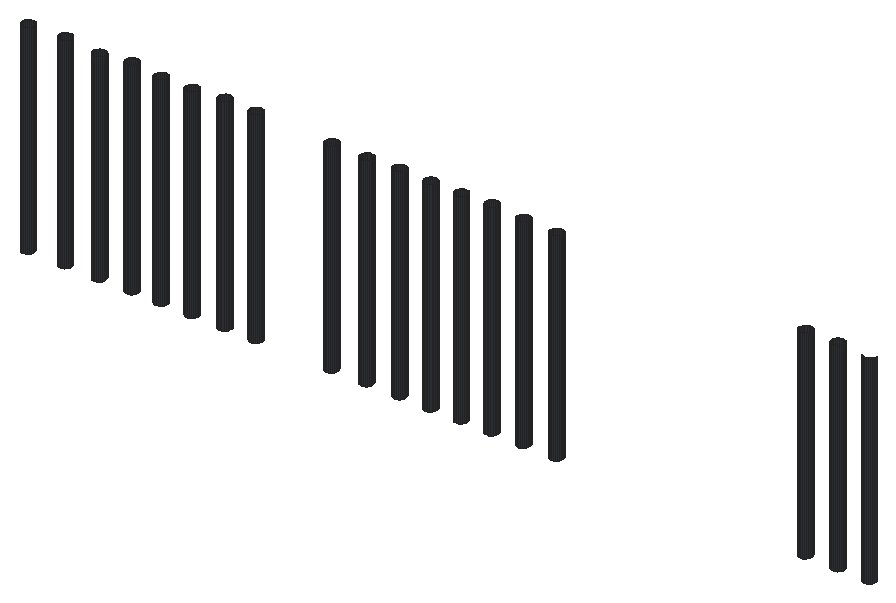
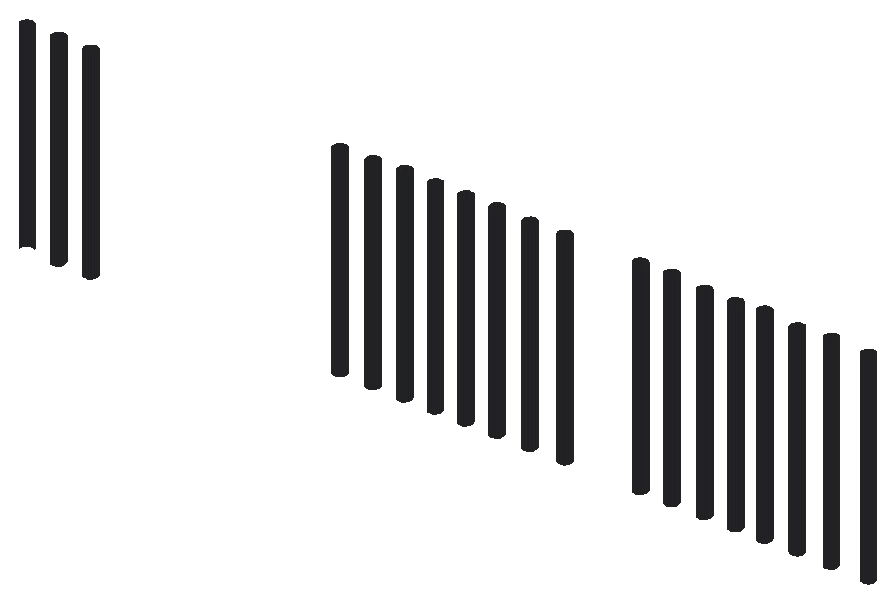
# SketchUp Ruby script. Lengths in inches.
U = 1.inch
M = Sketchup.active_model
def pt(a) = Geom::Point3d.new(a.map { |v| v * U })
def face(e, loops, mat)
  f = e.add_face(loops[0].map { |a| pt(a) })
  loops[1..].each { |l| e.add_face(l.map { |a| pt(a) }).erase! }
  f.material = f.back_material = mat if mat
  f
end
# faces: each face lists its corners as indices into pts; further lists are holes
def faces(e, pts, list, mat = nil) = list.each { |f| face(e, (f[0].is_a?(Array) ? f : [f]).map { |l| l.map { |i| pts[i] } }, mat) }
# xy, xz, yz: faces in a plane at the given z, y or x. An outline is a flat list of corners, or four numbers for a rectangle; further outlines are holes
def ring(l) = l.size == 4 ? [[l[0], l[1]], [l[2], l[1]], [l[2], l[3]], [l[0], l[3]]] : l.each_slice(2).to_a
def flat(e, list, mat, &to3) = list.each { |f| face(e, (f[0].is_a?(Array) ? f : [f]).map { |l| ring(l).map { |u, v| to3.(u, v) } }, mat) }
def xy(e, z, list, mat = nil) = flat(e, list, mat) { |x, y| [x, y, z] }
def xz(e, y, list, mat = nil) = flat(e, list, mat) { |x, z| [x, y, z] }
def yz(e, x, list, mat = nil) = flat(e, list, mat) { |y, z| [x, y, z] }
def lines(e, pts, list) = list.each { |a, b| e.add_line(pt(pts[a]), pt(pts[b])) }
# prism: a flat outline (further loops are holes) pulled along v
def prism(e, loops, v, mat = nil)
  f = face(e, loops, mat); d = Geom::Vector3d.new(v.map { |x| x * U })
  f.pushpull(f.normal.samedirection?(d) ? d.length : -d.length)
end
def box(e, o, s, mat = nil) = prism(e, [[o, [o[0] + s[0], o[1], o[2]], [o[0] + s[0], o[1] + s[1], o[2]], [o[0], o[1] + s[1], o[2]]]], [0, 0, s[2]], mat)
def at(x, y, z, deg = 0) = Geom::Transformation.translation(pt([x, y, z])) * Geom::Transformation.rotation(ORIGIN, Z_AXIS, deg.degrees)
def axes(o, x, y, z) = Geom::Transformation.new([*x, 0, *y, 0, *z, 0, *pt(o).to_a, 1])
def part(name) = M.definitions.add(name)
# library, detail: a bought-in or finely detailed component or shape, given as its bounding box
def library(name, o, s) = part(name).tap { |d| box(d.entities, o, s) }
def detail(e, o, s) = box(e.add_group.entities, o, s)
def put(e, d, t, mat = nil) = e.add_instance(d, t).tap { |i| i.material = mat if mat }
def group(e, t, mat = nil) = e.add_group.tap { |g| g.transformation = t; g.material = mat if mat }.entities
root = M.entities
M.materials.add("[Formica Laminate Dark]1").color = [50, 53, 60]
xy(root,29.875,[[1934.18,55.58,1931.67,55.72,1929.29,56.51,1927.18,57.89,1925.51,59.76,1924.38,62.01,1923.87,64.47,1924.01,66.98,1924.8,69.36,1926.18,71.46,1928.05,73.14,1930.29,74.27,1932.75,74.78,1935.26,74.64,1937.65,73.85,1939.75,72.47,1941.42,70.6,1942.55,68.35,1943.07,65.89,1942.92,63.38,1942.14,61,1940.76,58.9,1938.88,57.22,1936.64,56.09],[1991.49,55.58,1988.98,55.72,1986.6,56.51,1984.5,57.89,1982.82,59.76,1981.69,62.01,1981.18,64.47,1981.32,66.98,1982.11,69.36,1983.49,71.46,1985.36,73.14,1987.61,74.27,1990.07,74.78,1992.58,74.64,1994.96,73.85,1997.0625,72.47,1998.74,70.6,1999.87,68.35,2000.38,65.89,2000.24,63.38,1999.45,61,1998.07,58.9,1996.2,57.22,1993.95,56.09],[2044.37,55.58,2041.86,55.72,2039.47,56.51,2037.37,57.89,2035.7,59.76,2034.57,62.01,2034.06,64.47,2034.2,66.98,2034.99,69.36,2036.36,71.46,2038.24,73.14,2040.48,74.27,2042.94,74.78,2045.45,74.64,2047.84,73.85,2049.9375,72.47,2051.61,70.6,2052.74,68.35,2053.25,65.89,2053.11,63.38,2052.32,61,2050.95,58.9,2049.07,57.22,2046.83,56.09],[2094.55,55.58,2092.05,55.72,2089.66,56.51,2087.56,57.89,2085.89,59.76,2084.76,62.01,2084.24,64.47,2084.39,66.98,2085.17,69.36,2086.55,71.46,2088.43,73.14,2090.67,74.27,2093.13,74.78,2095.64,74.64,2098.02,73.85,2100.125,72.47,2101.8,70.6,2102.93,68.35,2103.44,65.89,2103.3,63.38,2102.51,61,2101.13,58.9,2099.26,57.22,2097.01,56.09],[2404.12,55.58,2401.61,55.72,2399.22,56.51,2397.12,57.89,2395.45,59.76,2394.32,62.01,2393.81,64.47,2393.95,66.98,2394.74,69.36,2396.11,71.46,2397.99,73.14,2400.23,74.27,2402.69,74.78,2405.2,74.64,2407.59,73.85,2409.6875,72.47,2411.36,70.6,2412.49,68.35,2413,65.89,2412.86,63.38,2412.07,61,2410.7,58.9,2408.82,57.22,2406.58,56.09],
  [2458.12,55.58,2455.61,55.72,2453.22,56.51,2451.12,57.89,2449.45,59.76,2448.32,62.01,2447.81,64.47,2447.95,66.98,2448.74,69.36,2450.11,71.46,2451.99,73.14,2454.23,74.27,2456.69,74.78,2459.2,74.64,2461.59,73.85,2463.6875,72.47,2465.36,70.6,2466.49,68.35,2467,65.89,2466.86,63.38,2466.07,61,2464.7,58.9,2462.82,57.22,2460.58,56.09],[2604.55,55.58,2602.05,55.72,2599.66,56.51,2597.56,57.89,2595.89,59.76,2594.76,62.01,2594.24,64.47,2594.39,66.98,2595.17,69.36,2596.55,71.46,2598.43,73.14,2600.67,74.27,2603.13,74.78,2605.64,74.64,2608.02,73.85,2610.125,72.47,2611.8,70.6,2612.93,68.35,2613.44,65.89,2613.3,63.38,2612.51,61,2611.13,58.9,2609.26,57.22,2607.01,56.09],[2700.93,55.58,2698.42,55.72,2696.04,56.51,2693.93,57.89,2692.26,59.76,2691.13,62.01,2690.62,64.47,2690.76,66.98,2691.55,69.36,2692.93,71.46,2694.8,73.14,2697.04,74.27,2699.5,74.78,2702.01,74.64,2704.4,73.85,2706.5,72.47,2708.17,70.6,2709.3,68.35,2709.82,65.89,2709.67,63.38,2708.89,61,2707.51,58.9,2705.63,57.22,2703.39,56.09],[2752.12,55.58,2749.61,55.72,2747.22,56.51,2745.12,57.89,2743.45,59.76,2742.32,62.01,2741.81,64.47,2741.95,66.98,2742.74,69.36,2744.11,71.46,2745.99,73.14,2748.23,74.27,2750.69,74.78,2753.2,74.64,2755.59,73.85,2757.6875,72.47,2759.36,70.6,2760.49,68.35,2761,65.89,2760.86,63.38,2760.07,61,2758.7,58.9,2756.82,57.22,2754.58,56.09]])
p = [[1931.67,55.72,29.875],[1934.18,55.58,29.875],[1934.18,55.58,343.5],[1931.67,55.72,343.5],[1936.64,56.09,29.875],[1936.64,56.09,343.5],
  [1988.98,55.72,29.875],[1991.49,55.58,29.875],[1991.49,55.58,345.54],[1988.98,55.72,345.54],[1993.95,56.09,29.875],[1993.95,56.09,345.54],
  [2041.86,55.72,29.875],[2044.37,55.58,29.875],[2044.37,55.58,341.4375],[2041.86,55.72,341.4375],[2046.83,56.09,29.875],[2046.83,56.09,341.4375],
  [2092.05,55.72,29.875],[2094.55,55.58,29.875],[2094.55,55.58,347.25],[2092.05,55.72,347.25],[2097.01,56.09,29.875],[2097.01,56.09,347.25],
  [2137.48,55.72,29.875],[2139.99,55.58,29.875],[2139.99,55.58,342.8],[2137.48,55.72,342.8],[2142.45,56.09,29.875],[2142.45,56.09,342.8],
  [2185.48,55.72,29.875],[2187.99,55.58,29.875],[2187.99,55.58,343.0625],[2185.48,55.72,343.0625],[2190.45,56.09,29.875],[2190.45,56.09,343.0625],
  [2236.17,55.72,29.875],[2238.68,55.58,29.875],[2238.68,55.58,347.3125],[2236.17,55.72,347.3125],[2241.14,56.09,29.875],[2241.14,56.09,347.3125],
  [2284.48,55.72,29.875],[2286.99,55.58,29.875],[2286.99,55.58,346.125],[2284.48,55.72,346.125],[2289.45,56.09,29.875],[2289.45,56.09,346.125],
  [2401.61,55.72,29.875],[2404.12,55.58,29.875],[2404.12,55.58,343.625],[2401.61,55.72,343.625],[2406.58,56.09,29.875],[2406.58,56.09,343.625],
  [2455.61,55.72,29.875],[2458.12,55.58,29.875],[2458.12,55.58,342.8],[2455.61,55.72,342.8],[2460.58,56.09,29.875],[2460.58,56.09,342.8],
  [2506.42,55.72,29.875],[2508.93,55.58,29.875],[2508.93,55.58,345],[2506.42,55.72,345],[2511.39,56.09,29.875],[2511.39,56.09,345],
  [2554.98,55.72,29.875],[2557.49,55.58,29.875],[2557.49,55.58,344.25],[2554.98,55.72,344.25],[2559.95,56.09,29.875],[2559.95,56.09,344.25],
  [2602.05,55.72,29.875],[2604.55,55.58,29.875],[2604.55,55.58,344.375],[2602.05,55.72,344.375],[2607.01,56.09,29.875],[2607.01,56.09,344.375],
  [2649.42,55.72,29.875],[2651.93,55.58,29.875],[2651.93,55.58,346],[2649.42,55.72,346],[2654.39,56.09,29.875],[2654.39,56.09,346],
  [2698.42,55.72,29.875],[2700.93,55.58,29.875],[2700.93,55.58,342.8],[2698.42,55.72,342.8],[2703.39,56.09,29.875],[2703.39,56.09,342.8],
  [2749.61,55.72,29.875],[2752.12,55.58,29.875],[2752.12,55.58,341.625],[2749.61,55.72,341.625],[2754.58,56.09,29.875],[2754.58,56.09,341.625],
  [3135.36,55.72,29.875],[3137.87,55.58,29.875],[3137.87,55.58,342.54],[3135.36,55.72,342.54],[3140.33,56.09,29.875],[3140.33,56.09,342.54],
  [3185.48,55.72,29.875],[3187.99,55.58,29.875],[3187.99,55.58,342.54],[3185.48,55.72,342.54],[3190.45,56.09,29.875],[3190.45,56.09,342.54],
  [3234.42,55.72,29.875],[3236.93,55.58,29.875],[3236.93,55.58,342.54],[3234.42,55.72,342.54],[3239.39,56.09,29.875],[3239.39,56.09,342.54],
  [1929.29,56.51,29.875],[1929.29,56.51,343.5],[1986.6,56.51,29.875],[1986.6,56.51,345.54],[2039.47,56.51,29.875],[2039.47,56.51,341.4375],
  [2089.66,56.51,29.875],[2089.66,56.51,347.25],[2135.1,56.51,29.875],[2135.1,56.51,342.8],[2183.1,56.51,29.875],[2183.1,56.51,343.0625],
  [2233.79,56.51,29.875],[2233.79,56.51,347.3125],[2282.1,56.51,29.875],[2282.1,56.51,346.125],[2399.22,56.51,29.875],[2399.22,56.51,343.625],
  [2453.22,56.51,29.875],[2453.22,56.51,342.8],[2504.04,56.51,29.875],[2504.04,56.51,345],[2552.6,56.51,29.875],[2552.6,56.51,344.25],
  [2599.66,56.51,29.875],[2599.66,56.51,344.375],[2647.04,56.51,29.875],[2647.04,56.51,346],[2696.04,56.51,29.875],[2696.04,56.51,342.8],
  [2747.22,56.51,29.875],[2747.22,56.51,341.625],[3132.97,56.51,29.875],[3132.97,56.51,342.54],[3183.1,56.51,29.875],[3183.1,56.51,342.54],
  [3232.04,56.51,29.875],[3232.04,56.51,342.54],[1938.88,57.22,29.875],[1938.88,57.22,343.5],[1996.2,57.22,29.875],[1996.2,57.22,345.54],
  [2049.07,57.22,29.875],[2049.07,57.22,341.4375],[2099.26,57.22,29.875],[2099.26,57.22,347.25],[2144.7,57.22,29.875],[2144.7,57.22,342.8],
  [2192.7,57.22,29.875],[2192.7,57.22,343.0625],[2243.38,57.22,29.875],[2243.38,57.22,347.3125],[2291.7,57.22,29.875],[2291.7,57.22,346.125],
  [2408.82,57.22,29.875],[2408.82,57.22,343.625],[2462.82,57.22,29.875],[2462.82,57.22,342.8],[2513.63,57.22,29.875],[2513.63,57.22,345],
  [2562.2,57.22,29.875],[2562.2,57.22,344.25],[2609.26,57.22,29.875],[2609.26,57.22,344.375],[2656.63,57.22,29.875],[2656.63,57.22,346],
  [2705.63,57.22,29.875],[2705.63,57.22,342.8],[2756.82,57.22,29.875],[2756.82,57.22,341.625],[3142.57,57.22,29.875],[3142.57,57.22,342.54],
  [3192.7,57.22,29.875],[3192.7,57.22,342.54],[3241.63,57.22,29.875],[3241.63,57.22,342.54],[1927.18,57.89,29.875],[1927.18,57.89,343.5],
  [1984.5,57.89,29.875],[1984.5,57.89,345.54],[2037.37,57.89,29.875],[2037.37,57.89,341.4375],[2087.56,57.89,29.875],[2087.56,57.89,347.25],
  [2133,57.89,29.875],[2133,57.89,342.8],[2181,57.89,29.875],[2181,57.89,343.0625],[2231.68,57.89,29.875],[2231.68,57.89,347.3125],
  [2280,57.89,29.875],[2280,57.89,346.125],[2397.12,57.89,29.875],[2397.12,57.89,343.625],[2451.12,57.89,29.875],[2451.12,57.89,342.8],
  [2501.93,57.89,29.875],[2501.93,57.89,345],[2550.5,57.89,29.875],[2550.5,57.89,344.25],[2597.56,57.89,29.875],[2597.56,57.89,344.375],
  [2644.93,57.89,29.875],[2644.93,57.89,346],[2693.93,57.89,29.875],[2693.93,57.89,342.8],[2745.12,57.89,29.875],[2745.12,57.89,341.625],
  [3130.87,57.89,29.875],[3130.87,57.89,342.54],[3181,57.89,29.875],[3181,57.89,342.54],[3229.93,57.89,29.875],[3229.93,57.89,342.54],
  [1940.76,58.9,29.875],[1940.76,58.9,343.5],[1998.07,58.9,29.875],[1998.07,58.9,345.54],[2050.95,58.9,29.875],[2050.95,58.9,341.4375],
  [2101.13,58.9,29.875],[2101.13,58.9,347.25],[2146.57,58.9,29.875],[2146.57,58.9,342.8],[2194.57,58.9,29.875],[2194.57,58.9,343.0625],
  [2245.26,58.9,29.875],[2245.26,58.9,347.3125],[2293.57,58.9,29.875],[2293.57,58.9,346.125],[2410.7,58.9,29.875],[2410.7,58.9,343.625],
  [2464.7,58.9,29.875],[2464.7,58.9,342.8],[2515.51,58.9,29.875],[2515.51,58.9,345],[2564.07,58.9,29.875],[2564.07,58.9,344.25],
  [2611.13,58.9,29.875],[2611.13,58.9,344.375],[2658.51,58.9,29.875],[2658.51,58.9,346],[2707.51,58.9,29.875],[2707.51,58.9,342.8],
  [2758.7,58.9,29.875],[2758.7,58.9,341.625],[3144.45,58.9,29.875],[3144.45,58.9,342.54],[3194.57,58.9,29.875],[3194.57,58.9,342.54],
  [3243.51,58.9,29.875],[3243.51,58.9,342.54],[1925.51,59.76,29.875],[1925.51,59.76,343.5],[1982.82,59.76,29.875],[1982.82,59.76,345.54],
  [2035.7,59.76,29.875],[2035.7,59.76,341.4375],[2085.89,59.76,29.875],[2085.89,59.76,347.25],[2131.32,59.76,29.875],[2131.32,59.76,342.8],
  [2179.32,59.76,29.875],[2179.32,59.76,343.0625],[2230.01,59.76,29.875],[2230.01,59.76,347.3125],[2278.32,59.76,29.875],[2278.32,59.76,346.125],
  [2395.45,59.76,29.875],[2395.45,59.76,343.625],[2449.45,59.76,29.875],[2449.45,59.76,342.8],[2500.26,59.76,29.875],[2500.26,59.76,345],
  [2548.82,59.76,29.875],[2548.82,59.76,344.25],[2595.89,59.76,29.875],[2595.89,59.76,344.375],[2643.26,59.76,29.875],[2643.26,59.76,346],
  [2692.26,59.76,29.875],[2692.26,59.76,342.8],[2743.45,59.76,29.875],[2743.45,59.76,341.625],[3129.2,59.76,29.875],[3129.2,59.76,342.54],
  [3179.32,59.76,29.875],[3179.32,59.76,342.54],[1942.14,61,29.875],[1942.14,61,343.5],[1999.45,61,29.875],[1999.45,61,345.54],
  [2052.32,61,29.875],[2052.32,61,341.4375],[2102.51,61,29.875],[2102.51,61,347.25],[2147.95,61,29.875],[2147.95,61,342.8],
  [2195.95,61,29.875],[2195.95,61,343.0625],[2246.64,61,29.875],[2246.64,61,347.3125],[2294.95,61,29.875],[2294.95,61,346.125],
  [2412.07,61,29.875],[2412.07,61,343.625],[2466.07,61,29.875],[2466.07,61,342.8],[2516.89,61,29.875],[2516.89,61,345],
  [2565.45,61,29.875],[2565.45,61,344.25],[2612.51,61,29.875],[2612.51,61,344.375],[2659.89,61,29.875],[2659.89,61,346],
  [2708.89,61,29.875],[2708.89,61,342.8],[2760.07,61,29.875],[2760.07,61,341.625],[3145.82,61,29.875],[3145.82,61,342.54],
  [3195.95,61,29.875],[3195.95,61,342.54],[3244.89,61,29.875],[3244.89,61,342.54],[1924.38,62.01,29.875],[1924.38,62.01,343.5],
  [1981.69,62.01,29.875],[1981.69,62.01,345.54],[2034.57,62.01,29.875],[2034.57,62.01,341.4375],[2084.76,62.01,29.875],[2084.76,62.01,347.25],
  [2130.19,62.01,29.875],[2130.19,62.01,342.8],[2178.19,62.01,29.875],[2178.19,62.01,343.0625],[2228.88,62.01,29.875],[2228.88,62.01,347.3125],
  [2277.19,62.01,29.875],[2277.19,62.01,346.125],[2394.32,62.01,29.875],[2394.32,62.01,343.625],[2448.32,62.01,29.875],[2448.32,62.01,342.8],
  [2499.13,62.01,29.875],[2499.13,62.01,345],[2547.69,62.01,29.875],[2547.69,62.01,344.25],[2594.76,62.01,29.875],[2594.76,62.01,344.375],
  [2642.13,62.01,29.875],[2642.13,62.01,346],[2691.13,62.01,29.875],[2691.13,62.01,342.8],[2742.32,62.01,29.875],[2742.32,62.01,341.625],
  [3128.07,62.01,29.875],[3128.07,62.01,342.54],[3178.19,62.01,29.875],[3178.19,62.01,342.54],[1942.92,63.38,29.875],[1942.92,63.38,343.5],
  [2000.24,63.38,29.875],[2000.24,63.38,345.54],[2053.11,63.38,29.875],[2053.11,63.38,341.4375],[2103.3,63.38,29.875],[2103.3,63.38,347.25],
  [2148.74,63.38,29.875],[2148.74,63.38,342.8],[2196.74,63.38,29.875],[2196.74,63.38,343.0625],[2247.42,63.38,29.875],[2247.42,63.38,347.3125],
  [2295.74,63.38,29.875],[2295.74,63.38,346.125],[2412.86,63.38,29.875],[2412.86,63.38,343.625],[2466.86,63.38,29.875],[2466.86,63.38,342.8],
  [2517.67,63.38,29.875],[2517.67,63.38,345],[2566.24,63.38,29.875],[2566.24,63.38,344.25],[2613.3,63.38,29.875],[2613.3,63.38,344.375],
  [2660.67,63.38,29.875],[2660.67,63.38,346],[2709.67,63.38,29.875],[2709.67,63.38,342.8],[2760.86,63.38,29.875],[2760.86,63.38,341.625],
  [3146.61,63.38,29.875],[3146.61,63.38,342.54],[3196.74,63.38,29.875],[3196.74,63.38,342.54],[3245.67,63.38,29.875],[3245.67,63.38,342.54],
  [1923.87,64.47,29.875],[1923.87,64.47,343.5],[1981.18,64.47,29.875],[1981.18,64.47,345.54],[2034.06,64.47,29.875],[2034.06,64.47,341.4375],
  [2084.24,64.47,29.875],[2084.24,64.47,347.25],[2129.68,64.47,29.875],[2129.68,64.47,342.8],[2177.68,64.47,29.875],[2177.68,64.47,343.0625],
  [2228.37,64.47,29.875],[2228.37,64.47,347.3125],[2276.68,64.47,29.875],[2276.68,64.47,346.125],[2393.81,64.47,29.875],[2393.81,64.47,343.625],
  [2447.81,64.47,29.875],[2447.81,64.47,342.8],[2498.62,64.47,29.875],[2498.62,64.47,345],[2547.18,64.47,29.875],[2547.18,64.47,344.25],
  [2594.24,64.47,29.875],[2594.24,64.47,344.375],[2641.62,64.47,29.875],[2641.62,64.47,346],[2690.62,64.47,29.875],[2690.62,64.47,342.8],
  [2741.81,64.47,29.875],[2741.81,64.47,341.625],[3127.56,64.47,29.875],[3127.56,64.47,342.54],[3177.68,64.47,29.875],[3177.68,64.47,342.54],
  [1943.07,65.89,29.875],[1943.07,65.89,343.5],[2000.38,65.89,29.875],[2000.38,65.89,345.54],[2053.25,65.89,29.875],[2053.25,65.89,341.4375],
  [2103.44,65.89,29.875],[2103.44,65.89,347.25],[2148.88,65.89,29.875],[2148.88,65.89,342.8],[2196.88,65.89,29.875],[2196.88,65.89,343.0625],
  [2247.57,65.89,29.875],[2247.57,65.89,347.3125],[2295.88,65.89,29.875],[2295.88,65.89,346.125],[2413,65.89,29.875],[2413,65.89,343.625],
  [2467,65.89,29.875],[2467,65.89,342.8],[2517.82,65.89,29.875],[2517.82,65.89,345],[2566.38,65.89,29.875],[2566.38,65.89,344.25],
  [2613.44,65.89,29.875],[2613.44,65.89,344.375],[2660.82,65.89,29.875],[2660.82,65.89,346],[2709.82,65.89,29.875],[2709.82,65.89,342.8],
  [2761,65.89,29.875],[2761,65.89,341.625],[3146.75,65.89,29.875],[3146.75,65.89,342.54],[3196.88,65.89,29.875],[3196.88,65.89,342.54],
  [3245.82,65.89,29.875],[3245.82,65.89,342.54],[1924.01,66.98,29.875],[1924.01,66.98,343.5],[1981.32,66.98,29.875],[1981.32,66.98,345.54],
  [2034.2,66.98,29.875],[2034.2,66.98,341.4375],[2084.39,66.98,29.875],[2084.39,66.98,347.25],[2129.82,66.98,29.875],[2129.82,66.98,342.8],
  [2177.82,66.98,29.875],[2177.82,66.98,343.0625],[2228.51,66.98,29.875],[2228.51,66.98,347.3125],[2276.82,66.98,29.875],[2276.82,66.98,346.125],
  [2393.95,66.98,29.875],[2393.95,66.98,343.625],[2447.95,66.98,29.875],[2447.95,66.98,342.8],[2498.76,66.98,29.875],[2498.76,66.98,345],
  [2547.32,66.98,29.875],[2547.32,66.98,344.25],[2594.39,66.98,29.875],[2594.39,66.98,344.375],[2641.76,66.98,29.875],[2641.76,66.98,346],
  [2690.76,66.98,29.875],[2690.76,66.98,342.8],[2741.95,66.98,29.875],[2741.95,66.98,341.625],[3127.7,66.98,29.875],[3127.7,66.98,342.54],
  [3177.82,66.98,29.875],[3177.82,66.98,342.54],[1942.55,68.35,29.875],[1942.55,68.35,343.5],[1999.87,68.35,29.875],[1999.87,68.35,345.54],
  [2052.74,68.35,29.875],[2052.74,68.35,341.4375],[2102.93,68.35,29.875],[2102.93,68.35,347.25],[2148.37,68.35,29.875],[2148.37,68.35,342.8],
  [2196.37,68.35,29.875],[2196.37,68.35,343.0625],[2247.05,68.35,29.875],[2247.05,68.35,347.3125],[2295.37,68.35,29.875],[2295.37,68.35,346.125],
  [2412.49,68.35,29.875],[2412.49,68.35,343.625],[2466.49,68.35,29.875],[2466.49,68.35,342.8],[2517.3,68.35,29.875],[2517.3,68.35,345],
  [2565.87,68.35,29.875],[2565.87,68.35,344.25],[2612.93,68.35,29.875],[2612.93,68.35,344.375],[2660.3,68.35,29.875],[2660.3,68.35,346],
  [2709.3,68.35,29.875],[2709.3,68.35,342.8],[2760.49,68.35,29.875],[2760.49,68.35,341.625],[3146.24,68.35,29.875],[3146.24,68.35,342.54],
  [3196.37,68.35,29.875],[3196.37,68.35,342.54],[1924.8,69.36,29.875],[1924.8,69.36,343.5],[1982.11,69.36,29.875],[1982.11,69.36,345.54],
  [2034.99,69.36,29.875],[2034.99,69.36,341.4375],[2085.17,69.36,29.875],[2085.17,69.36,347.25],[2130.61,69.36,29.875],[2130.61,69.36,342.8],
  [2178.61,69.36,29.875],[2178.61,69.36,343.0625],[2229.3,69.36,29.875],[2229.3,69.36,347.3125],[2277.61,69.36,29.875],[2277.61,69.36,346.125],
  [2394.74,69.36,29.875],[2394.74,69.36,343.625],[2448.74,69.36,29.875],[2448.74,69.36,342.8],[2499.55,69.36,29.875],[2499.55,69.36,345],
  [2548.11,69.36,29.875],[2548.11,69.36,344.25],[2595.17,69.36,29.875],[2595.17,69.36,344.375],[2642.55,69.36,29.875],[2642.55,69.36,346],
  [2691.55,69.36,29.875],[2691.55,69.36,342.8],[2742.74,69.36,29.875],[2742.74,69.36,341.625],[3128.49,69.36,29.875],[3128.49,69.36,342.54],
  [3178.61,69.36,29.875],[3178.61,69.36,342.54],[1941.42,70.6,29.875],[1941.42,70.6,343.5],[1998.74,70.6,29.875],[1998.74,70.6,345.54],
  [2051.61,70.6,29.875],[2051.61,70.6,341.4375],[2101.8,70.6,29.875],[2101.8,70.6,347.25],[2147.24,70.6,29.875],[2147.24,70.6,342.8],
  [2195.24,70.6,29.875],[2195.24,70.6,343.0625],[2245.92,70.6,29.875],[2245.92,70.6,347.3125],[2294.24,70.6,29.875],[2294.24,70.6,346.125],
  [2411.36,70.6,29.875],[2411.36,70.6,343.625],[2465.36,70.6,29.875],[2465.36,70.6,342.8],[2516.17,70.6,29.875],[2516.17,70.6,345],
  [2564.74,70.6,29.875],[2564.74,70.6,344.25],[2611.8,70.6,29.875],[2611.8,70.6,344.375],[2659.17,70.6,29.875],[2659.17,70.6,346],
  [2708.17,70.6,29.875],[2708.17,70.6,342.8],[2759.36,70.6,29.875],[2759.36,70.6,341.625],[3145.11,70.6,29.875],[3145.11,70.6,342.54],
  [3195.24,70.6,29.875],[3195.24,70.6,342.54],[1926.18,71.46,29.875],[1926.18,71.46,343.5],[1983.49,71.46,29.875],[1983.49,71.46,345.54],
  [2036.36,71.46,29.875],[2036.36,71.46,341.4375],[2086.55,71.46,29.875],[2086.55,71.46,347.25],[2131.99,71.46,29.875],[2131.99,71.46,342.8],
  [2179.99,71.46,29.875],[2179.99,71.46,343.0625],[2230.68,71.46,29.875],[2230.68,71.46,347.3125],[2278.99,71.46,29.875],[2278.99,71.46,346.125],
  [2396.11,71.46,29.875],[2396.11,71.46,343.625],[2450.11,71.46,29.875],[2450.11,71.46,342.8],[2500.93,71.46,29.875],[2500.93,71.46,345],
  [2549.49,71.46,29.875],[2549.49,71.46,344.25],[2596.55,71.46,29.875],[2596.55,71.46,344.375],[2643.93,71.46,29.875],[2643.93,71.46,346],
  [2692.93,71.46,29.875],[2692.93,71.46,342.8],[2744.11,71.46,29.875],[2744.11,71.46,341.625],[3129.86,71.46,29.875],[3129.86,71.46,342.54],
  [3179.99,71.46,29.875],[3179.99,71.46,342.54],[1939.75,72.47,29.875],[1939.75,72.47,343.5],[1997.0625,72.47,29.875],[1997.0625,72.47,345.54],
  [2049.9375,72.47,29.875],[2049.9375,72.47,341.4375],[2100.125,72.47,29.875],[2100.125,72.47,347.25],[2145.5625,72.47,29.875],[2145.5625,72.47,342.8],
  [2193.5625,72.47,29.875],[2193.5625,72.47,343.0625],[2244.25,72.47,29.875],[2244.25,72.47,347.3125],[2292.5625,72.47,29.875],[2292.5625,72.47,346.125],
  [2409.6875,72.47,29.875],[2409.6875,72.47,343.625],[2463.6875,72.47,29.875],[2463.6875,72.47,342.8],[2514.5,72.47,29.875],[2514.5,72.47,345],
  [2563.0625,72.47,29.875],[2563.0625,72.47,344.25],[2610.125,72.47,29.875],[2610.125,72.47,344.375],[2657.5,72.47,29.875],[2657.5,72.47,346],
  [2706.5,72.47,29.875],[2706.5,72.47,342.8],[2757.6875,72.47,29.875],[2757.6875,72.47,341.625],[3143.4375,72.47,29.875],[3143.4375,72.47,342.54],
  [3193.5625,72.47,29.875],[3193.5625,72.47,342.54],[1928.05,73.14,29.875],[1928.05,73.14,343.5],[1985.36,73.14,29.875],[1985.36,73.14,345.54],
  [2038.24,73.14,29.875],[2038.24,73.14,341.4375],[2088.43,73.14,29.875],[2088.43,73.14,347.25],[2133.86,73.14,29.875],[2133.86,73.14,342.8],
  [2181.86,73.14,29.875],[2181.86,73.14,343.0625],[2232.55,73.14,29.875],[2232.55,73.14,347.3125],[2280.86,73.14,29.875],[2280.86,73.14,346.125],
  [2397.99,73.14,29.875],[2397.99,73.14,343.625],[2451.99,73.14,29.875],[2451.99,73.14,342.8],[2502.8,73.14,29.875],[2502.8,73.14,345],
  [2551.36,73.14,29.875],[2551.36,73.14,344.25],[2598.43,73.14,29.875],[2598.43,73.14,344.375],[2645.8,73.14,29.875],[2645.8,73.14,346],
  [2694.8,73.14,29.875],[2694.8,73.14,342.8],[2745.99,73.14,29.875],[2745.99,73.14,341.625],[3131.74,73.14,29.875],[3131.74,73.14,342.54],
  [3181.86,73.14,29.875],[3181.86,73.14,342.54],[1937.65,73.85,29.875],[1937.65,73.85,343.5],[1994.96,73.85,29.875],[1994.96,73.85,345.54],
  [2047.84,73.85,29.875],[2047.84,73.85,341.4375],[2098.02,73.85,29.875],[2098.02,73.85,347.25],[2143.46,73.85,29.875],[2143.46,73.85,342.8],
  [2191.46,73.85,29.875],[2191.46,73.85,343.0625],[2242.15,73.85,29.875],[2242.15,73.85,347.3125],[2290.46,73.85,29.875],[2290.46,73.85,346.125],
  [2407.59,73.85,29.875],[2407.59,73.85,343.625],[2461.59,73.85,29.875],[2461.59,73.85,342.8],[2512.4,73.85,29.875],[2512.4,73.85,345],
  [2560.96,73.85,29.875],[2560.96,73.85,344.25],[2608.02,73.85,29.875],[2608.02,73.85,344.375],[2655.4,73.85,29.875],[2655.4,73.85,346],
  [2704.4,73.85,29.875],[2704.4,73.85,342.8],[2755.59,73.85,29.875],[2755.59,73.85,341.625],[3141.34,73.85,29.875],[3141.34,73.85,342.54],
  [3191.46,73.85,29.875],[3191.46,73.85,342.54],[1930.29,74.27,29.875],[1930.29,74.27,343.5],[1987.61,74.27,29.875],[1987.61,74.27,345.54],
  [2040.48,74.27,29.875],[2040.48,74.27,341.4375],[2090.67,74.27,29.875],[2090.67,74.27,347.25],[2136.11,74.27,29.875],[2136.11,74.27,342.8],
  [2184.11,74.27,29.875],[2184.11,74.27,343.0625],[2234.79,74.27,29.875],[2234.79,74.27,347.3125],[2283.11,74.27,29.875],[2283.11,74.27,346.125],
  [2400.23,74.27,29.875],[2400.23,74.27,343.625],[2454.23,74.27,29.875],[2454.23,74.27,342.8],[2505.04,74.27,29.875],[2505.04,74.27,345],
  [2553.61,74.27,29.875],[2553.61,74.27,344.25],[2600.67,74.27,29.875],[2600.67,74.27,344.375],[2648.04,74.27,29.875],[2648.04,74.27,346],
  [2697.04,74.27,29.875],[2697.04,74.27,342.8],[2748.23,74.27,29.875],[2748.23,74.27,341.625],[3133.98,74.27,29.875],[3133.98,74.27,342.54],
  [3184.11,74.27,29.875],[3184.11,74.27,342.54],[1935.26,74.64,29.875],[1935.26,74.64,343.5],[1992.58,74.64,29.875],[1992.58,74.64,345.54],
  [2045.45,74.64,29.875],[2045.45,74.64,341.4375],[2095.64,74.64,29.875],[2095.64,74.64,347.25],[2141.08,74.64,29.875],[2141.08,74.64,342.8],
  [2189.08,74.64,29.875],[2189.08,74.64,343.0625],[2239.76,74.64,29.875],[2239.76,74.64,347.3125],[2288.08,74.64,29.875],[2288.08,74.64,346.125],
  [2405.2,74.64,29.875],[2405.2,74.64,343.625],[2459.2,74.64,29.875],[2459.2,74.64,342.8],[2510.01,74.64,29.875],[2510.01,74.64,345],
  [2558.58,74.64,29.875],[2558.58,74.64,344.25],[2605.64,74.64,29.875],[2605.64,74.64,344.375],[2653.01,74.64,29.875],[2653.01,74.64,346],
  [2702.01,74.64,29.875],[2702.01,74.64,342.8],[2753.2,74.64,29.875],[2753.2,74.64,341.625],[3138.95,74.64,29.875],[3138.95,74.64,342.54],
  [3189.08,74.64,29.875],[3189.08,74.64,342.54],[1932.75,74.78,29.875],[1932.75,74.78,343.5],[1990.07,74.78,29.875],[1990.07,74.78,345.54],
  [2042.94,74.78,29.875],[2042.94,74.78,341.4375],[2093.13,74.78,29.875],[2093.13,74.78,347.25],[2138.57,74.78,29.875],[2138.57,74.78,342.8],
  [2186.57,74.78,29.875],[2186.57,74.78,343.0625],[2237.25,74.78,29.875],[2237.25,74.78,347.3125],[2285.57,74.78,29.875],[2285.57,74.78,346.125],
  [2402.69,74.78,29.875],[2402.69,74.78,343.625],[2456.69,74.78,29.875],[2456.69,74.78,342.8],[2507.5,74.78,29.875],[2507.5,74.78,345],
  [2556.07,74.78,29.875],[2556.07,74.78,344.25],[2603.13,74.78,29.875],[2603.13,74.78,344.375],[2650.5,74.78,29.875],[2650.5,74.78,346],
  [2699.5,74.78,29.875],[2699.5,74.78,342.8],[2750.69,74.78,29.875],[2750.69,74.78,341.625],[3136.44,74.78,29.875],[3136.44,74.78,342.54],
  [3186.57,74.78,29.875],[3186.57,74.78,342.54]]
faces(root,p,[[0,1,2,3],[1,4,5,2],[6,7,8,9],[7,10,11,8],[12,13,14,15],[13,16,17,14],[18,19,20,21],[19,22,23,20],
  [24,25,26,27],[25,28,29,26],[30,31,32,33],[31,34,35,32],[36,37,38,39],[37,40,41,38],[42,43,44,45],[43,46,47,44],
  [48,49,50,51],[49,52,53,50],[54,55,56,57],[55,58,59,56],[60,61,62,63],[61,64,65,62],[66,67,68,69],[67,70,71,68],
  [72,73,74,75],[73,76,77,74],[78,79,80,81],[79,82,83,80],[84,85,86,87],[85,88,89,86],[90,91,92,93],[91,94,95,92],
  [96,97,98,99],[97,100,101,98],[102,103,104,105],[103,106,107,104],[108,109,110,111],[109,112,113,110],[114,0,3,115],[116,6,9,117],
  [118,12,15,119],[120,18,21,121],[122,24,27,123],[124,30,33,125],[126,36,39,127],[128,42,45,129],[130,48,51,131],[132,54,57,133],
  [134,60,63,135],[136,66,69,137],[138,72,75,139],[140,78,81,141],[142,84,87,143],[144,90,93,145],[146,96,99,147],[148,102,105,149],
  [150,108,111,151],[4,152,153,5],[10,154,155,11],[16,156,157,17],[22,158,159,23],[28,160,161,29],[34,162,163,35],[40,164,165,41],
  [46,166,167,47],[52,168,169,53],[58,170,171,59],[64,172,173,65],[70,174,175,71],[76,176,177,77],[82,178,179,83],[88,180,181,89],
  [94,182,183,95],[100,184,185,101],[106,186,187,107],[112,188,189,113],[190,114,115,191],[192,116,117,193],[194,118,119,195],[196,120,121,197],
  [198,122,123,199],[200,124,125,201],[202,126,127,203],[204,128,129,205],[206,130,131,207],[208,132,133,209],[210,134,135,211],[212,136,137,213],
  [214,138,139,215],[216,140,141,217],[218,142,143,219],[220,144,145,221],[222,146,147,223],[224,148,149,225],[226,150,151,227],[152,228,229,153],
  [154,230,231,155],[156,232,233,157],[158,234,235,159],[160,236,237,161],[162,238,239,163],[164,240,241,165],[166,242,243,167],[168,244,245,169],
  [170,246,247,171],[172,248,249,173],[174,250,251,175],[176,252,253,177],[178,254,255,179],[180,256,257,181],[182,258,259,183],[184,260,261,185],
  [186,262,263,187],[188,264,265,189],[266,190,191,267],[268,192,193,269],[270,194,195,271],[272,196,197,273],[274,198,199,275],[276,200,201,277],
  [278,202,203,279],[280,204,205,281],[282,206,207,283],[284,208,209,285],[286,210,211,287],[288,212,213,289],[290,214,215,291],[292,216,217,293],
  [294,218,219,295],[296,220,221,297],[298,222,223,299],[300,224,225,301],[228,302,303,229],[230,304,305,231],[232,306,307,233],[234,308,309,235],
  [236,310,311,237],[238,312,313,239],[240,314,315,241],[242,316,317,243],[244,318,319,245],[246,320,321,247],[248,322,323,249],[250,324,325,251],
  [252,326,327,253],[254,328,329,255],[256,330,331,257],[258,332,333,259],[260,334,335,261],[262,336,337,263],[264,338,339,265],[340,266,267,341],
  [342,268,269,343],[344,270,271,345],[346,272,273,347],[348,274,275,349],[350,276,277,351],[352,278,279,353],[354,280,281,355],[356,282,283,357],
  [358,284,285,359],[360,286,287,361],[362,288,289,363],[364,290,291,365],[366,292,293,367],[368,294,295,369],[370,296,297,371],[372,298,299,373],
  [374,300,301,375],[302,376,377,303],[304,378,379,305],[306,380,381,307],[308,382,383,309],[310,384,385,311],[312,386,387,313],[314,388,389,315],
  [316,390,391,317],[318,392,393,319],[320,394,395,321],[322,396,397,323],[324,398,399,325],[326,400,401,327],[328,402,403,329],[330,404,405,331],
  [332,406,407,333],[334,408,409,335],[336,410,411,337],[338,412,413,339],[414,340,341,415],[416,342,343,417],[418,344,345,419],[420,346,347,421],
  [422,348,349,423],[424,350,351,425],[426,352,353,427],[428,354,355,429],[430,356,357,431],[432,358,359,433],[434,360,361,435],[436,362,363,437],
  [438,364,365,439],[440,366,367,441],[442,368,369,443],[444,370,371,445],[446,372,373,447],[448,374,375,449],[376,450,451,377],[378,452,453,379],
  [380,454,455,381],[382,456,457,383],[384,458,459,385],[386,460,461,387],[388,462,463,389],[390,464,465,391],[392,466,467,393],[394,468,469,395],
  [396,470,471,397],[398,472,473,399],[400,474,475,401],[402,476,477,403],[404,478,479,405],[406,480,481,407],[408,482,483,409],[410,484,485,411],
  [412,486,487,413],[488,414,415,489],[490,416,417,491],[492,418,419,493],[494,420,421,495],[496,422,423,497],[498,424,425,499],[500,426,427,501],
  [502,428,429,503],[504,430,431,505],[506,432,433,507],[508,434,435,509],[510,436,437,511],[512,438,439,513],[514,440,441,515],[516,442,443,517],
  [518,444,445,519],[520,446,447,521],[522,448,449,523],[450,524,525,451],[452,526,527,453],[454,528,529,455],[456,530,531,457],[458,532,533,459],
  [460,534,535,461],[462,536,537,463],[464,538,539,465],[466,540,541,467],[468,542,543,469],[470,544,545,471],[472,546,547,473],[474,548,549,475],
  [476,550,551,477],[478,552,553,479],[480,554,555,481],[482,556,557,483],[484,558,559,485],[560,488,489,561],[562,490,491,563],[564,492,493,565],
  [566,494,495,567],[568,496,497,569],[570,498,499,571],[572,500,501,573],[574,502,503,575],[576,504,505,577],[578,506,507,579],[580,508,509,581],
  [582,510,511,583],[584,512,513,585],[586,514,515,587],[588,516,517,589],[590,518,519,591],[592,520,521,593],[594,522,523,595],[524,596,597,525],
  [526,598,599,527],[528,600,601,529],[530,602,603,531],[532,604,605,533],[534,606,607,535],[536,608,609,537],[538,610,611,539],[540,612,613,541],
  [542,614,615,543],[544,616,617,545],[546,618,619,547],[548,620,621,549],[550,622,623,551],[552,624,625,553],[554,626,627,555],[556,628,629,557],
  [558,630,631,559],[632,560,561,633],[634,562,563,635],[636,564,565,637],[638,566,567,639],[640,568,569,641],[642,570,571,643],[644,572,573,645],
  [646,574,575,647],[648,576,577,649],[650,578,579,651],[652,580,581,653],[654,582,583,655],[656,584,585,657],[658,586,587,659],[660,588,589,661],
  [662,590,591,663],[664,592,593,665],[666,594,595,667],[596,668,669,597],[598,670,671,599],[600,672,673,601],[602,674,675,603],[604,676,677,605],
  [606,678,679,607],[608,680,681,609],[610,682,683,611],[612,684,685,613],[614,686,687,615],[616,688,689,617],[618,690,691,619],[620,692,693,621],
  [622,694,695,623],[624,696,697,625],[626,698,699,627],[628,700,701,629],[630,702,703,631],[704,632,633,705],[706,634,635,707],[708,636,637,709],
  [710,638,639,711],[712,640,641,713],[714,642,643,715],[716,644,645,717],[718,646,647,719],[720,648,649,721],[722,650,651,723],[724,652,653,725],
  [726,654,655,727],[728,656,657,729],[730,658,659,731],[732,660,661,733],[734,662,663,735],[736,664,665,737],[738,666,667,739],[668,740,741,669],
  [670,742,743,671],[672,744,745,673],[674,746,747,675],[676,748,749,677],[678,750,751,679],[680,752,753,681],[682,754,755,683],[684,756,757,685],
  [686,758,759,687],[688,760,761,689],[690,762,763,691],[692,764,765,693],[694,766,767,695],[696,768,769,697],[698,770,771,699],[700,772,773,701],
  [702,774,775,703],[776,704,705,777],[778,706,707,779],[780,708,709,781],[782,710,711,783],[784,712,713,785],[786,714,715,787],[788,716,717,789],
  [790,718,719,791],[792,720,721,793],[794,722,723,795],[796,724,725,797],[798,726,727,799],[800,728,729,801],[802,730,731,803],[804,732,733,805],
  [806,734,735,807],[808,736,737,809],[810,738,739,811],[740,812,813,741],[742,814,815,743],[744,816,817,745],[746,818,819,747],[748,820,821,749],
  [750,822,823,751],[752,824,825,753],[754,826,827,755],[756,828,829,757],[758,830,831,759],[760,832,833,761],[762,834,835,763],[764,836,837,765],
  [766,838,839,767],[768,840,841,769],[770,842,843,771],[772,844,845,773],[774,846,847,775],[848,776,777,849],[850,778,779,851],[852,780,781,853],
  [854,782,783,855],[856,784,785,857],[858,786,787,859],[860,788,789,861],[862,790,791,863],[864,792,793,865],[866,794,795,867],[868,796,797,869],
  [870,798,799,871],[872,800,801,873],[874,802,803,875],[876,804,805,877],[878,806,807,879],[880,808,809,881],[882,810,811,883],[812,848,849,813],
  [814,850,851,815],[816,852,853,817],[818,854,855,819],[820,856,857,821],[822,858,859,823],[824,860,861,825],[826,862,863,827],[828,864,865,829],
  [830,866,867,831],[832,868,869,833],[834,870,871,835],[836,872,873,837],[838,874,875,839],[840,876,877,841],[842,878,879,843],[844,880,881,845],
  [846,882,883,847]],"[Formica Laminate Dark]1")
